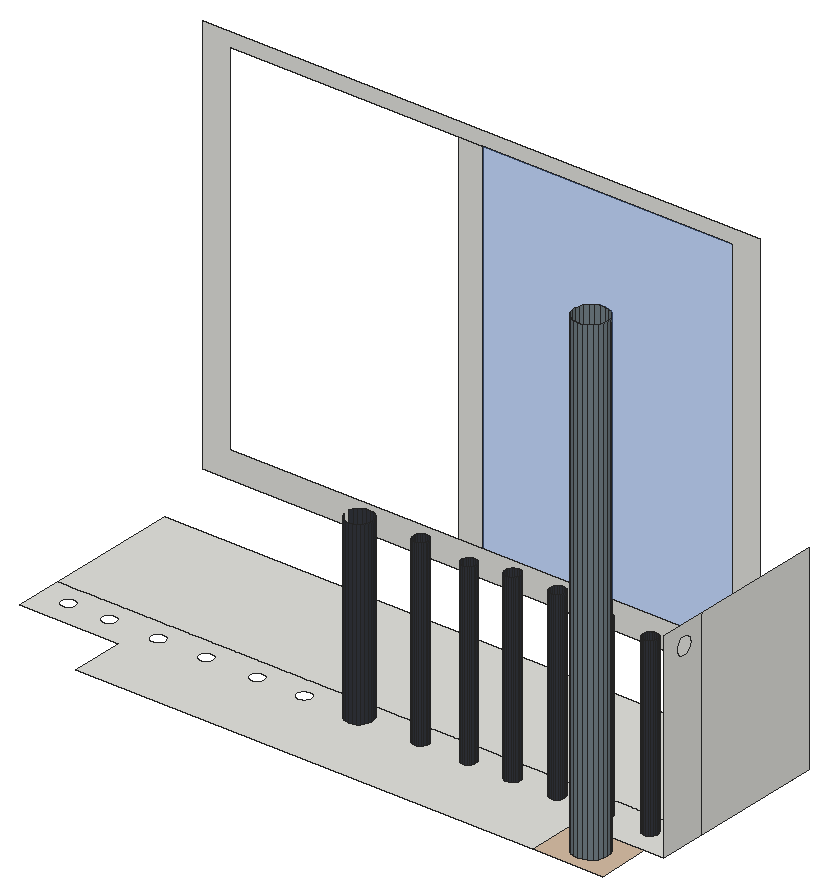
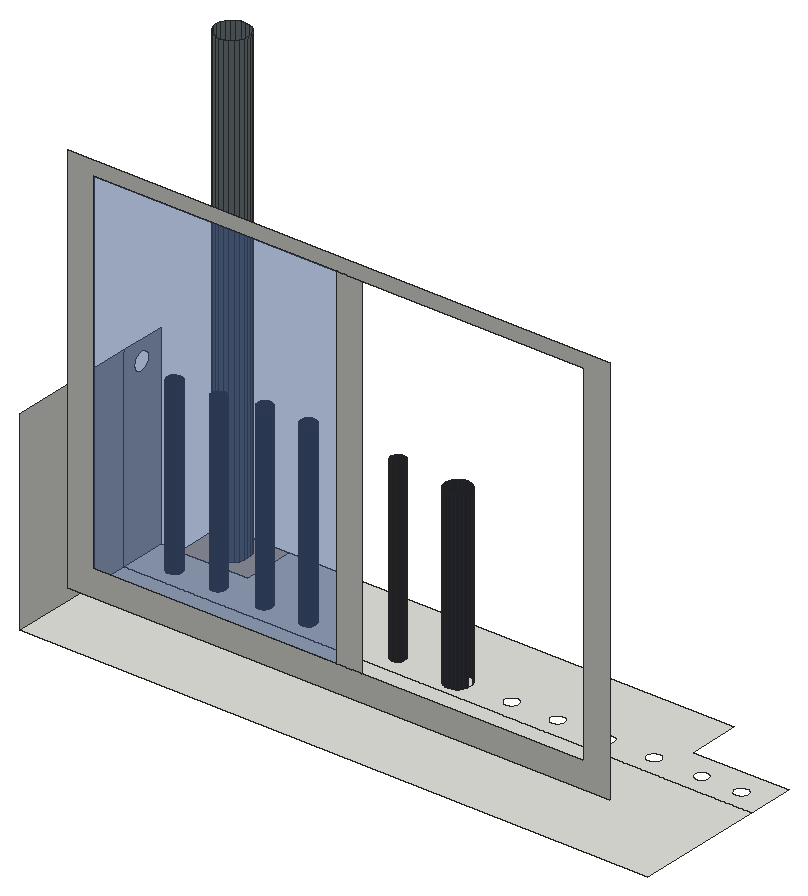
# SketchUp Ruby script. Lengths in inches.
U = 1.inch
M = Sketchup.active_model
def pt(a) = Geom::Point3d.new(a.map { |v| v * U })
def face(e, loops, mat)
  f = e.add_face(loops[0].map { |a| pt(a) })
  loops[1..].each { |l| e.add_face(l.map { |a| pt(a) }).erase! }
  f.material = f.back_material = mat if mat
  f
end
# faces: each face lists its corners as indices into pts; further lists are holes
def faces(e, pts, list, mat = nil) = list.each { |f| face(e, (f[0].is_a?(Array) ? f : [f]).map { |l| l.map { |i| pts[i] } }, mat) }
# xy, xz, yz: faces in a plane at the given z, y or x. An outline is a flat list of corners, or four numbers for a rectangle; further outlines are holes
def ring(l) = l.size == 4 ? [[l[0], l[1]], [l[2], l[1]], [l[2], l[3]], [l[0], l[3]]] : l.each_slice(2).to_a
def flat(e, list, mat, &to3) = list.each { |f| face(e, (f[0].is_a?(Array) ? f : [f]).map { |l| ring(l).map { |u, v| to3.(u, v) } }, mat) }
def xy(e, z, list, mat = nil) = flat(e, list, mat) { |x, y| [x, y, z] }
def xz(e, y, list, mat = nil) = flat(e, list, mat) { |x, z| [x, y, z] }
def yz(e, x, list, mat = nil) = flat(e, list, mat) { |y, z| [x, y, z] }
def lines(e, pts, list) = list.each { |a, b| e.add_line(pt(pts[a]), pt(pts[b])) }
# prism: a flat outline (further loops are holes) pulled along v
def prism(e, loops, v, mat = nil)
  f = face(e, loops, mat); d = Geom::Vector3d.new(v.map { |x| x * U })
  f.pushpull(f.normal.samedirection?(d) ? d.length : -d.length)
end
def box(e, o, s, mat = nil) = prism(e, [[o, [o[0] + s[0], o[1], o[2]], [o[0] + s[0], o[1] + s[1], o[2]], [o[0], o[1] + s[1], o[2]]]], [0, 0, s[2]], mat)
def at(x, y, z, deg = 0) = Geom::Transformation.translation(pt([x, y, z])) * Geom::Transformation.rotation(ORIGIN, Z_AXIS, deg.degrees)
def axes(o, x, y, z) = Geom::Transformation.new([*x, 0, *y, 0, *z, 0, *pt(o).to_a, 1])
def part(name) = M.definitions.add(name)
# library, detail: a bought-in or finely detailed component or shape, given as its bounding box
def library(name, o, s) = part(name).tap { |d| box(d.entities, o, s) }
def detail(e, o, s) = box(e.add_group.entities, o, s)
def put(e, d, t, mat = nil) = e.add_instance(d, t).tap { |i| i.material = mat if mat }
def group(e, t, mat = nil) = e.add_group.tap { |g| g.transformation = t; g.material = mat if mat }.entities
root = M.entities
M.materials.add("[Formica Laminate Dark]").color = [50, 53, 60]
M.materials.add("[Formica Laminate Light]").color = [213, 189, 164]
M.materials.add("[Formica Speckled Grey]").color = [112, 125, 132]
M.materials.add("[Translucent Glass Blue]").color = [85, 126, 201]
M.materials["[Translucent Glass Blue]"].alpha = 0.5
xy(root,272.93,[[[307.63,82.54,369.37,82.54,369.37,89.73,381.41,89.73,381.41,96.06,294.34,96.06,294.34,89.73,307.63,89.73],[337.23,91.64,336.78,91.7,336.36,91.875,335.99,92.15,335.72,92.51,335.54,92.9375,335.48,93.39,335.54,93.84,335.72,94.26,335.99,94.625,336.36,94.9,336.78,95.08,337.23,95.14,337.68,95.08,338.11,94.9,338.47,94.625,338.75,94.26,338.92,93.84,338.98,93.39,338.92,92.9375,338.75,92.51,338.47,92.15,338.11,91.875,337.68,91.7],[329.95,92.22,329.69,92.25,329.45,92.35,329.24,92.51,329.08,92.72,328.98,92.96,328.95,93.22,328.98,93.48,329.08,93.72,329.24,93.93,329.45,94.09,329.69,94.1875,329.95,94.22,330.21,94.1875,330.45,94.09,330.66,93.93,330.82,93.72,330.92,93.48,330.95,93.22,330.92,92.96,330.82,92.72,330.66,92.51,330.45,92.35,330.21,92.25],[323.57,92.22,323.32,92.25,323.07,92.35,322.87,92.51,322.71,92.72,322.61,92.96,322.57,93.22,322.61,93.48,322.71,93.72,322.87,93.93,323.07,94.09,323.32,94.1875,323.57,94.22,323.83,94.1875,324.07,94.09,324.28,93.93,324.44,93.72,324.54,93.48,324.57,93.22,324.54,92.96,324.44,92.72,324.28,92.51,324.07,92.35,323.83,92.25],[298.07,92.22,297.82,92.25,297.57,92.35,297.37,92.51,297.21,92.72,297.11,92.96,297.07,93.22,297.11,93.48,297.21,93.72,297.37,93.93,297.57,94.09,297.82,94.1875,298.07,94.22,298.33,94.1875,298.57,94.09,298.78,93.93,298.94,93.72,299.04,93.48,299.07,93.22,299.04,92.96,298.94,92.72,298.78,92.51,298.57,92.35,298.33,92.25],[303.57,92.22,303.32,92.25,303.07,92.35,302.87,92.51,302.71,92.72,302.61,92.96,302.57,93.22,302.61,93.48,302.71,93.72,302.87,93.93,303.07,94.09,303.32,94.1875,303.57,94.22,303.83,94.1875,304.07,94.09,304.28,93.93,304.44,93.72,304.54,93.48,304.57,93.22,304.54,92.96,304.44,92.72,304.28,92.51,304.07,92.35,303.83,92.25],[310.2,92.22,309.94,92.25,309.7,92.35,309.49,92.51,309.33,92.72,309.23,92.96,309.2,93.22,309.23,93.48,309.33,93.72,309.49,93.93,309.7,94.09,309.94,94.1875,310.2,94.22,310.46,94.1875,310.7,94.09,310.91,93.93,311.07,93.72,311.17,93.48,311.2,93.22,311.17,92.96,311.07,92.72,310.91,92.51,310.7,92.35,310.46,92.25],[316.7,92.22,316.44,92.25,316.2,92.35,315.99,92.51,315.83,92.72,315.73,92.96,315.7,93.22,315.73,93.48,315.83,93.72,315.99,93.93,316.2,94.09,316.44,94.1875,316.7,94.22,316.96,94.1875,317.2,94.09,317.41,93.93,317.57,93.72,317.67,93.48,317.7,93.22,317.67,92.96,317.57,92.72,317.41,92.51,317.2,92.35,316.96,92.25],[345.7,92.22,345.44,92.25,345.2,92.35,344.99,92.51,344.83,92.72,344.73,92.96,344.7,93.22,344.73,93.48,344.83,93.72,344.99,93.93,345.2,94.09,345.44,94.1875,345.7,94.22,345.96,94.1875,346.2,94.09,346.41,93.93,346.57,93.72,346.67,93.48,346.7,93.22,346.67,92.96,346.57,92.72,346.41,92.51,346.2,92.35,345.96,92.25],[376.7,92.22,376.44,92.25,376.2,92.35,375.99,92.51,375.83,92.72,375.73,92.96,375.7,93.22,375.73,93.48,375.83,93.72,375.99,93.93,376.2,94.09,376.44,94.1875,376.7,94.22,376.96,94.1875,377.2,94.09,377.41,93.93,377.57,93.72,377.67,93.48,377.7,93.22,377.67,92.96,377.57,92.72,377.41,92.51,377.2,92.35,376.96,92.25],[352.2,92.22,351.94,92.25,351.7,92.35,351.49,92.51,351.33,92.72,351.23,92.96,351.2,93.22,351.23,93.48,351.33,93.72,351.49,93.93,351.7,94.09,351.94,94.1875,352.2,94.22,352.46,94.1875,352.7,94.09,352.91,93.93,353.07,93.72,353.17,93.48,353.2,93.22,353.17,92.96,353.07,92.72,352.91,92.51,352.7,92.35,352.46,92.25],[370.57,92.22,370.32,92.25,370.07,92.35,369.87,92.51,369.71,92.72,369.61,92.96,369.57,93.22,369.61,93.48,369.71,93.72,369.87,93.93,370.07,94.09,370.32,94.1875,370.57,94.22,370.83,94.1875,371.07,94.09,371.28,93.93,371.44,93.72,371.54,93.48,371.57,93.22,371.54,92.96,371.44,92.72,371.28,92.51,371.07,92.35,370.83,92.25],[358.14,92.22,357.88,92.25,357.64,92.35,357.43,92.51,357.27,92.72,357.17,92.96,357.14,93.22,357.17,93.48,357.27,93.72,357.43,93.93,357.64,94.09,357.88,94.1875,358.14,94.22,358.4,94.1875,358.64,94.09,358.84,93.93,359,93.72,359.1,93.48,359.14,93.22,359.1,92.96,359,92.72,358.84,92.51,358.64,92.35,358.4,92.25],[364.2,92.22,363.94,92.25,363.7,92.35,363.49,92.51,363.33,92.72,363.23,92.96,363.2,93.22,363.23,93.48,363.33,93.72,363.49,93.93,363.7,94.09,363.94,94.1875,364.2,94.22,364.46,94.1875,364.7,94.09,364.91,93.93,365.07,93.72,365.17,93.48,365.2,93.22,365.17,92.96,365.07,92.72,364.91,92.51,364.7,92.35,364.46,92.25]],[374.29,84.01,373.71,84.08,373.16,84.31,372.7,84.67,372.34,85.13,372.12,85.67,372.04,86.26,372.12,86.84,372.34,87.38,372.7,87.85,373.16,88.21,373.71,88.43,374.29,88.51,374.87,88.43,375.41,88.21,375.88,87.85,376.24,87.38,376.46,86.84,376.54,86.26,376.46,85.67,376.24,85.13,375.88,84.67,375.41,84.31,374.87,84.08],[337.23,91.64,336.78,91.7,336.36,91.875,335.99,92.15,335.72,92.51,335.54,92.9375,335.48,93.39,335.54,93.84,335.72,94.26,335.99,94.625,336.36,94.9,336.78,95.08,337.23,95.14,337.68,95.08,338.11,94.9,338.47,94.625,338.75,94.26,338.92,93.84,338.98,93.39,338.92,92.9375,338.75,92.51,338.47,92.15,338.11,91.875,337.68,91.7],[345.7,92.22,345.44,92.25,345.2,92.35,344.99,92.51,344.83,92.72,344.73,92.96,344.7,93.22,344.73,93.48,344.83,93.72,344.99,93.93,345.2,94.09,345.44,94.1875,345.7,94.22,345.96,94.1875,346.2,94.09,346.41,93.93,346.57,93.72,346.67,93.48,346.7,93.22,346.67,92.96,346.57,92.72,346.41,92.51,346.2,92.35,345.96,92.25],[352.2,92.22,351.94,92.25,351.7,92.35,351.49,92.51,351.33,92.72,351.23,92.96,351.2,93.22,351.23,93.48,351.33,93.72,351.49,93.93,351.7,94.09,351.94,94.1875,352.2,94.22,352.46,94.1875,352.7,94.09,352.91,93.93,353.07,93.72,353.17,93.48,353.2,93.22,353.17,92.96,353.07,92.72,352.91,92.51,352.7,92.35,352.46,92.25],
  [358.14,92.22,357.88,92.25,357.64,92.35,357.43,92.51,357.27,92.72,357.17,92.96,357.14,93.22,357.17,93.48,357.27,93.72,357.43,93.93,357.64,94.09,357.88,94.1875,358.14,94.22,358.4,94.1875,358.64,94.09,358.84,93.93,359,93.72,359.1,93.48,359.14,93.22,359.1,92.96,359,92.72,358.84,92.51,358.64,92.35,358.4,92.25],[364.2,92.22,363.94,92.25,363.7,92.35,363.49,92.51,363.33,92.72,363.23,92.96,363.2,93.22,363.23,93.48,363.33,93.72,363.49,93.93,363.7,94.09,363.94,94.1875,364.2,94.22,364.46,94.1875,364.7,94.09,364.91,93.93,365.07,93.72,365.17,93.48,365.2,93.22,365.17,92.96,365.07,92.72,364.91,92.51,364.7,92.35,364.46,92.25],[370.57,92.22,370.32,92.25,370.07,92.35,369.87,92.51,369.71,92.72,369.61,92.96,369.57,93.22,369.61,93.48,369.71,93.72,369.87,93.93,370.07,94.09,370.32,94.1875,370.57,94.22,370.83,94.1875,371.07,94.09,371.28,93.93,371.44,93.72,371.54,93.48,371.57,93.22,371.54,92.96,371.44,92.72,371.28,92.51,371.07,92.35,370.83,92.25],[376.7,92.22,376.44,92.25,376.2,92.35,375.99,92.51,375.83,92.72,375.73,92.96,375.7,93.22,375.73,93.48,375.83,93.72,375.99,93.93,376.2,94.09,376.44,94.1875,376.7,94.22,376.96,94.1875,377.2,94.09,377.41,93.93,377.57,93.72,377.67,93.48,377.7,93.22,377.67,92.96,377.57,92.72,377.41,92.51,377.2,92.35,376.96,92.25],[294.34,96.06,381.41,114.1]])
xy(root,272.93,[[[369.37,82.54,378.82,89.73],[374.29,84.01,373.71,84.08,373.16,84.31,372.7,84.67,372.34,85.13,372.12,85.67,372.04,86.26,372.12,86.84,372.34,87.38,372.7,87.85,373.16,88.21,373.71,88.43,374.29,88.51,374.87,88.43,375.41,88.21,375.88,87.85,376.24,87.38,376.46,86.84,376.54,86.26,376.46,85.67,376.24,85.13,375.88,84.67,375.41,84.31,374.87,84.08]]],"[Formica Laminate Light]")
xz(root,114.1,[[[299.6,280.54,374.79,334.91],[303.24,284.18,371.15,332.96]],[334.08,284.18,337.4375,332.96]])
xz(root,114.1,[[337.4375,284.18,371.15,332.96]],"[Translucent Glass Blue]")
yz(root,381.41,[[[89.73,272.93,96.06,299.8],[93.0625,295.87,93.39,295.91,93.6875,296.04,93.95,296.23,94.15,296.49,94.27,296.79,94.3125,297.12,94.27,297.44,94.15,297.74,93.95,298,93.6875,298.2,93.39,298.33,93.0625,298.37,92.74,298.33,92.4375,298.2,92.18,298,91.98,297.74,91.86,297.44,91.8125,297.12,91.86,296.79,91.98,296.49,92.18,296.23,92.4375,296.04,92.74,295.91]],[96.06,272.93,114.1,299.8]])
p = [[373.71,84.08,272.93],[374.29,84.01,272.93],[374.29,84.01,337.71],[373.71,84.08,337.71],[374.87,84.08,272.93],[374.87,84.08,337.71],
  [373.16,84.31,272.93],[373.16,84.31,337.71],[375.41,84.31,272.93],[375.41,84.31,337.71],[372.7,84.67,272.93],[372.7,84.67,337.71],
  [375.88,84.67,272.93],[375.88,84.67,337.71],[372.34,85.13,272.93],[372.34,85.13,337.71],[376.24,85.13,272.93],[376.24,85.13,337.71],
  [372.12,85.67,272.93],[372.12,85.67,337.71],[376.46,85.67,272.93],[376.46,85.67,337.71],[372.04,86.26,272.93],[372.04,86.26,337.71],
  [376.54,86.26,272.93],[376.54,86.26,337.71],[372.12,86.84,272.93],[372.12,86.84,337.71],[376.46,86.84,272.93],[376.46,86.84,337.71],
  [372.34,87.38,272.93],[372.34,87.38,337.71],[376.24,87.38,272.93],[376.24,87.38,337.71],[372.7,87.85,272.93],[372.7,87.85,337.71],
  [375.88,87.85,272.93],[375.88,87.85,337.71],[373.16,88.21,272.93],[373.16,88.21,337.71],[375.41,88.21,272.93],[375.41,88.21,337.71],
  [373.71,88.43,272.93],[373.71,88.43,337.71],[374.87,88.43,272.93],[374.87,88.43,337.71],[374.29,88.51,272.93],[374.29,88.51,337.71],
  [336.78,91.7,272.93],[337.23,91.64,272.93],[337.23,91.64,297.11],[336.78,91.7,297.11],[337.68,91.7,272.93],[337.68,91.7,297.11],
  [336.36,91.875,272.93],[336.36,91.875,297.11],[338.11,91.875,272.93],[338.11,91.875,297.11],[335.99,92.15,272.93],[335.99,92.15,297.11],
  [338.47,92.15,272.93],[338.47,92.15,297.11],[335.72,92.51,272.93],[335.72,92.51,297.11],[338.75,92.51,272.93],[338.75,92.51,297.11],
  [345.44,92.25,272.93],[345.7,92.22,272.93],[345.7,92.22,297.55],[345.44,92.25,297.55],[345.96,92.25,272.93],[345.96,92.25,297.55],
  [351.94,92.25,272.93],[352.2,92.22,272.93],[352.2,92.22,296.93],[351.94,92.25,296.93],[352.46,92.25,272.93],[352.46,92.25,296.93],
  [357.88,92.25,272.93],[358.14,92.22,272.93],[358.14,92.22,297.74],[357.88,92.25,297.74],[358.4,92.25,272.93],[358.4,92.25,297.74],
  [363.94,92.25,272.93],[364.2,92.22,272.93],[364.2,92.22,297.74],[363.94,92.25,297.74],[364.46,92.25,272.93],[364.46,92.25,297.74],
  [370.32,92.25,272.93],[370.57,92.22,272.93],[370.57,92.22,296.68],[370.32,92.25,296.68],[370.83,92.25,272.93],[370.83,92.25,296.68],
  [376.44,92.25,272.93],[376.7,92.22,272.93],[376.7,92.22,296.55],[376.44,92.25,296.55],[376.96,92.25,272.93],[376.96,92.25,296.55],
  [345.2,92.35,272.93],[345.2,92.35,297.55],[346.2,92.35,272.93],[346.2,92.35,297.55],[351.7,92.35,272.93],[351.7,92.35,296.93],
  [352.7,92.35,272.93],[352.7,92.35,296.93],[357.64,92.35,272.93],[357.64,92.35,297.74],[358.64,92.35,272.93],[358.64,92.35,297.74],
  [363.7,92.35,272.93],[363.7,92.35,297.74],[364.7,92.35,272.93],[364.7,92.35,297.74],[370.07,92.35,272.93],[370.07,92.35,296.68],
  [371.07,92.35,272.93],[371.07,92.35,296.68],[376.2,92.35,272.93],[376.2,92.35,296.55],[377.2,92.35,272.93],[377.2,92.35,296.55],
  [344.99,92.51,272.93],[344.99,92.51,297.55],[346.41,92.51,272.93],[346.41,92.51,297.55],[351.49,92.51,272.93],[351.49,92.51,296.93],
  [352.91,92.51,272.93],[352.91,92.51,296.93],[357.43,92.51,272.93],[357.43,92.51,297.74],[358.84,92.51,272.93],[358.84,92.51,297.74],
  [363.49,92.51,272.93],[363.49,92.51,297.74],[364.91,92.51,272.93],[364.91,92.51,297.74],[369.87,92.51,272.93],[369.87,92.51,296.68],
  [371.28,92.51,272.93],[371.28,92.51,296.68],[375.99,92.51,272.93],[375.99,92.51,296.55],[377.41,92.51,272.93],[377.41,92.51,296.55],
  [335.54,92.9375,272.93],[335.54,92.9375,297.11],[338.92,92.9375,272.93],[338.92,92.9375,297.11],[344.83,92.72,272.93],[344.83,92.72,297.55],
  [346.57,92.72,272.93],[346.57,92.72,297.55],[351.33,92.72,272.93],[351.33,92.72,296.93],[353.07,92.72,272.93],[353.07,92.72,296.93],
  [357.27,92.72,272.93],[357.27,92.72,297.74],[359,92.72,272.93],[359,92.72,297.74],[363.33,92.72,272.93],[363.33,92.72,297.74],
  [365.07,92.72,272.93],[365.07,92.72,297.74],[369.71,92.72,272.93],[369.71,92.72,296.68],[371.44,92.72,272.93],[371.44,92.72,296.68],
  [375.83,92.72,272.93],[375.83,92.72,296.55],[377.57,92.72,272.93],[377.57,92.72,296.55],[344.73,92.96,272.93],[344.73,92.96,297.55],
  [346.67,92.96,272.93],[346.67,92.96,297.55],[351.23,92.96,272.93],[351.23,92.96,296.93],[353.17,92.96,272.93],[353.17,92.96,296.93],
  [357.17,92.96,272.93],[357.17,92.96,297.74],[359.1,92.96,272.93],[359.1,92.96,297.74],[363.23,92.96,272.93],[363.23,92.96,297.74],
  [365.17,92.96,272.93],[365.17,92.96,297.74],[369.61,92.96,272.93],[369.61,92.96,296.68],[371.54,92.96,272.93],[371.54,92.96,296.68],
  [375.73,92.96,272.93],[375.73,92.96,296.55],[377.67,92.96,272.93],[377.67,92.96,296.55],[338.98,93.39,272.93],[338.98,93.39,297.11],
  [344.7,93.22,272.93],[344.7,93.22,297.55],[346.7,93.22,272.93],[346.7,93.22,297.55],[351.2,93.22,272.93],[351.2,93.22,296.93],
  [353.2,93.22,272.93],[353.2,93.22,296.93],[357.14,93.22,272.93],[357.14,93.22,297.74],[359.14,93.22,272.93],[359.14,93.22,297.74],
  [363.2,93.22,272.93],[363.2,93.22,297.74],[365.2,93.22,272.93],[365.2,93.22,297.74],[369.57,93.22,272.93],[369.57,93.22,296.68],
  [371.57,93.22,272.93],[371.57,93.22,296.68],[375.7,93.22,272.93],[375.7,93.22,296.55],[377.7,93.22,272.93],[377.7,93.22,296.55],
  [344.73,93.48,272.93],[344.73,93.48,297.55],[346.67,93.48,272.93],[346.67,93.48,297.55],[351.23,93.48,272.93],[351.23,93.48,296.93],
  [353.17,93.48,272.93],[353.17,93.48,296.93],[357.17,93.48,272.93],[357.17,93.48,297.74],[359.1,93.48,272.93],[359.1,93.48,297.74],
  [363.23,93.48,272.93],[363.23,93.48,297.74],[365.17,93.48,272.93],[365.17,93.48,297.74],[369.61,93.48,272.93],[369.61,93.48,296.68],
  [371.54,93.48,272.93],[371.54,93.48,296.68],[375.73,93.48,272.93],[375.73,93.48,296.55],[377.67,93.48,272.93],[377.67,93.48,296.55],
  [338.92,93.84,272.93],[338.92,93.84,297.11],[344.83,93.72,272.93],[344.83,93.72,297.55],[346.57,93.72,272.93],[346.57,93.72,297.55],
  [351.33,93.72,272.93],[351.33,93.72,296.93],[353.07,93.72,272.93],[353.07,93.72,296.93],[357.27,93.72,272.93],[357.27,93.72,297.74],
  [359,93.72,272.93],[359,93.72,297.74],[363.33,93.72,272.93],[363.33,93.72,297.74],[365.07,93.72,272.93],[365.07,93.72,297.74],
  [369.71,93.72,272.93],[369.71,93.72,296.68],[371.44,93.72,272.93],[371.44,93.72,296.68],[375.83,93.72,272.93],[375.83,93.72,296.55],
  [377.57,93.72,272.93],[377.57,93.72,296.55],[344.99,93.93,272.93],[344.99,93.93,297.55],[346.41,93.93,272.93],[346.41,93.93,297.55],
  [351.49,93.93,272.93],[351.49,93.93,296.93],[352.91,93.93,272.93],[352.91,93.93,296.93],[357.43,93.93,272.93],[357.43,93.93,297.74],
  [358.84,93.93,272.93],[358.84,93.93,297.74],[363.49,93.93,272.93],[363.49,93.93,297.74],[364.91,93.93,272.93],[364.91,93.93,297.74],
  [369.87,93.93,272.93],[369.87,93.93,296.68],[371.28,93.93,272.93],[371.28,93.93,296.68],[375.99,93.93,272.93],[375.99,93.93,296.55],
  [377.41,93.93,272.93],[377.41,93.93,296.55],[335.72,94.26,272.93],[335.54,93.84,272.93],[335.54,93.84,297.11],[335.72,94.26,297.11],
  [338.75,94.26,272.93],[338.75,94.26,297.11],[345.2,94.09,272.93],[345.2,94.09,297.55],[346.2,94.09,272.93],[346.2,94.09,297.55],
  [351.7,94.09,272.93],[351.7,94.09,296.93],[352.7,94.09,272.93],[352.7,94.09,296.93],[357.64,94.09,272.93],[357.64,94.09,297.74],
  [358.64,94.09,272.93],[358.64,94.09,297.74],[363.7,94.09,272.93],[363.7,94.09,297.74],[364.7,94.09,272.93],[364.7,94.09,297.74],
  [370.07,94.09,272.93],[370.07,94.09,296.68],[371.07,94.09,272.93],[371.07,94.09,296.68],[376.2,94.09,272.93],[376.2,94.09,296.55],
  [377.2,94.09,272.93],[377.2,94.09,296.55],[345.44,94.1875,272.93],[345.44,94.1875,297.55],[345.96,94.1875,272.93],[345.96,94.1875,297.55],
  [351.94,94.1875,272.93],[351.94,94.1875,296.93],[352.46,94.1875,272.93],[352.46,94.1875,296.93],[357.88,94.1875,272.93],[357.78,94.15,297.74],
  [357.88,94.1875,297.74],[358.4,94.1875,272.93],[358.4,94.1875,297.74],[358.49,94.15,297.74],[363.94,94.1875,272.93],[363.94,94.1875,297.74],
  [364.46,94.1875,272.93],[364.46,94.1875,297.74],[370.32,94.1875,272.93],[370.32,94.1875,296.68],[370.83,94.1875,272.93],[370.83,94.1875,296.68],
  [376.44,94.1875,272.93],[376.44,94.1875,296.55],[376.96,94.1875,272.93],[376.96,94.1875,296.55],[345.7,94.22,272.93],[345.7,94.22,297.55],
  [352.2,94.22,272.93],[352.2,94.22,296.93],[358.14,94.22,272.93],[358.14,94.22,297.74],[364.2,94.22,272.93],[364.2,94.22,297.74],
  [370.57,94.22,272.93],[370.57,94.22,296.68],[376.7,94.22,272.93],[376.7,94.22,296.55],[335.99,94.625,272.93],[335.99,94.625,297.11],
  [338.47,94.625,272.93],[338.47,94.625,297.11],[336.36,94.9,272.93],[336.36,94.9,297.11],[338.11,94.9,272.93],[338.11,94.9,297.11],
  [336.78,95.08,272.93],[336.78,95.08,297.11],[337.68,95.08,272.93],[337.68,95.08,297.11],[337.23,95.14,272.93],[337.23,95.14,297.11]]
faces(root,p,[[0,1,2,3],[1,4,5,2],[6,0,3,7],[4,8,9,5],[10,6,7,11],[8,12,13,9],[14,10,11,15],[12,16,17,13],
  [18,14,15,19],[16,20,21,17],[22,18,19,23],[20,24,25,21],[26,22,23,27],[24,28,29,25],[30,26,27,31],[28,32,33,29],
  [34,30,31,35],[32,36,37,33],[38,34,35,39],[36,40,41,37],[42,38,39,43],[40,44,45,41],[46,42,43,47],[44,46,47,45]],"[Formica Speckled Grey]")
faces(root,p,[[48,49,50,51],[49,52,53,50],[54,48,51,55],[52,56,57,53],[58,54,55,59],[56,60,61,57],[62,58,59,63],[60,64,65,61],
  [66,67,68,69],[67,70,71,68],[72,73,74,75],[73,76,77,74],[78,79,80,81],[79,82,83,80],[84,85,86,87],[85,88,89,86],
  [90,91,92,93],[91,94,95,92],[96,97,98,99],[97,100,101,98],[102,66,69,103],[70,104,105,71],[106,72,75,107],[76,108,109,77],
  [110,78,81,111],[82,112,113,83],[114,84,87,115],[88,116,117,89],[118,90,93,119],[94,120,121,95],[122,96,99,123],[100,124,125,101],
  [126,102,103,127],[104,128,129,105],[130,106,107,131],[108,132,133,109],[134,110,111,135],[112,136,137,113],[138,114,115,139],[116,140,141,117],
  [142,118,119,143],[120,144,145,121],[146,122,123,147],[124,148,149,125],[150,62,63,151],[64,152,153,65],[154,126,127,155],[128,156,157,129],
  [158,130,131,159],[132,160,161,133],[162,134,135,163],[136,164,165,137],[166,138,139,167],[140,168,169,141],[170,142,143,171],[144,172,173,145],
  [174,146,147,175],[148,176,177,149],[178,154,155,179],[156,180,181,157],[182,158,159,183],[160,184,185,161],[186,162,163,187],[164,188,189,165],
  [190,166,167,191],[168,192,193,169],[194,170,171,195],[172,196,197,173],[198,174,175,199],[176,200,201,177],[152,202,203,153],[204,178,179,205],
  [180,206,207,181],[208,182,183,209],[184,210,211,185],[212,186,187,213],[188,214,215,189],[216,190,191,217],[192,218,219,193],[220,194,195,221],
  [196,222,223,197],[224,198,199,225],[200,226,227,201],[228,204,205,229],[206,230,231,207],[232,208,209,233],[210,234,235,211],[236,212,213,237],
  [214,238,239,215],[240,216,217,241],[218,242,243,219],[244,220,221,245],[222,246,247,223],[248,224,225,249],[226,250,251,227],[202,252,253,203],
  [254,228,229,255],[230,256,257,231],[258,232,233,259],[234,260,261,235],[262,236,237,263],[238,264,265,239],[266,240,241,267],[242,268,269,243],
  [270,244,245,271],[246,272,273,247],[274,248,249,275],[250,276,277,251],[278,254,255,279],[256,280,281,257],[282,258,259,283],[260,284,285,261],
  [286,262,263,287],[264,288,289,265],[290,266,267,291],[268,292,293,269],[294,270,271,295],[272,296,297,273],[298,274,275,299],[276,300,301,277],
  [302,303,304,305],[252,306,307,253],[308,278,279,309],[280,310,311,281],[312,282,283,313],[284,314,315,285],[316,286,287,317],[288,318,319,289],
  [320,290,291,321],[292,322,323,293],[324,294,295,325],[296,326,327,297],[328,298,299,329],[300,330,331,301],[332,308,309,333],[310,334,335,311],
  [336,312,313,337],[314,338,339,315],[340,316,317,341,342],[318,343,344,345,319],[346,320,321,347],[322,348,349,323],[350,324,325,351],[326,352,353,327],
  [354,328,329,355],[330,356,357,331],[358,332,333,359],[334,358,359,335],[360,336,337,361],[338,360,361,339],[362,340,342,363],[343,362,363,344],
  [364,346,347,365],[348,364,365,349],[366,350,351,367],[352,366,367,353],[368,354,355,369],[356,368,369,357],[370,302,305,371],[306,372,373,307],
  [374,370,371,375],[372,376,377,373],[378,374,375,379],[376,380,381,377],[382,378,379,383],[380,382,383,381]],"[Formica Laminate Dark]")
